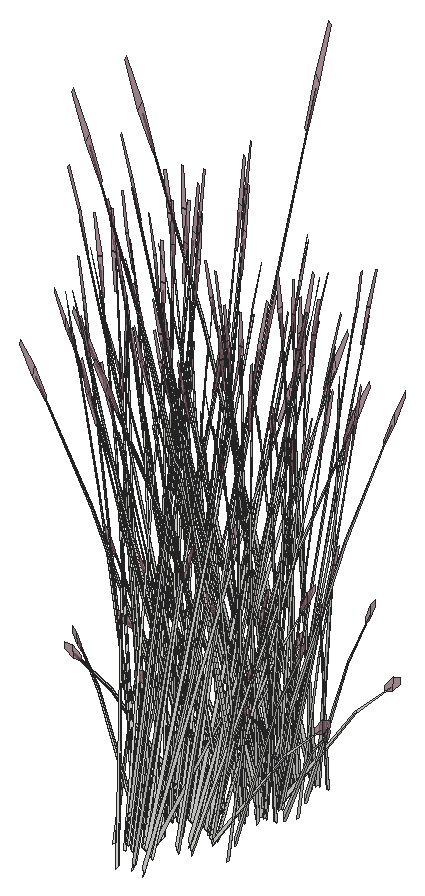
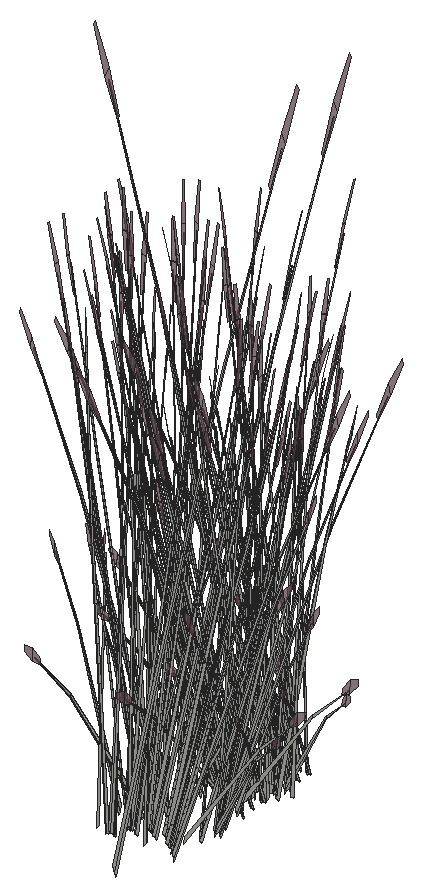
# SketchUp Ruby script. Lengths in inches.
U = 1.inch
M = Sketchup.active_model
def pt(a) = Geom::Point3d.new(a.map { |v| v * U })
def face(e, loops, mat)
  f = e.add_face(loops[0].map { |a| pt(a) })
  loops[1..].each { |l| e.add_face(l.map { |a| pt(a) }).erase! }
  f.material = f.back_material = mat if mat
  f
end
# faces: each face lists its corners as indices into pts; further lists are holes
def faces(e, pts, list, mat = nil) = list.each { |f| face(e, (f[0].is_a?(Array) ? f : [f]).map { |l| l.map { |i| pts[i] } }, mat) }
# xy, xz, yz: faces in a plane at the given z, y or x. An outline is a flat list of corners, or four numbers for a rectangle; further outlines are holes
def ring(l) = l.size == 4 ? [[l[0], l[1]], [l[2], l[1]], [l[2], l[3]], [l[0], l[3]]] : l.each_slice(2).to_a
def flat(e, list, mat, &to3) = list.each { |f| face(e, (f[0].is_a?(Array) ? f : [f]).map { |l| ring(l).map { |u, v| to3.(u, v) } }, mat) }
def xy(e, z, list, mat = nil) = flat(e, list, mat) { |x, y| [x, y, z] }
def xz(e, y, list, mat = nil) = flat(e, list, mat) { |x, z| [x, y, z] }
def yz(e, x, list, mat = nil) = flat(e, list, mat) { |y, z| [x, y, z] }
def lines(e, pts, list) = list.each { |a, b| e.add_line(pt(pts[a]), pt(pts[b])) }
# prism: a flat outline (further loops are holes) pulled along v
def prism(e, loops, v, mat = nil)
  f = face(e, loops, mat); d = Geom::Vector3d.new(v.map { |x| x * U })
  f.pushpull(f.normal.samedirection?(d) ? d.length : -d.length)
end
def box(e, o, s, mat = nil) = prism(e, [[o, [o[0] + s[0], o[1], o[2]], [o[0] + s[0], o[1] + s[1], o[2]], [o[0], o[1] + s[1], o[2]]]], [0, 0, s[2]], mat)
def at(x, y, z, deg = 0) = Geom::Transformation.translation(pt([x, y, z])) * Geom::Transformation.rotation(ORIGIN, Z_AXIS, deg.degrees)
def axes(o, x, y, z) = Geom::Transformation.new([*x, 0, *y, 0, *z, 0, *pt(o).to_a, 1])
def part(name) = M.definitions.add(name)
# library, detail: a bought-in or finely detailed component or shape, given as its bounding box
def library(name, o, s) = part(name).tap { |d| box(d.entities, o, s) }
def detail(e, o, s) = box(e.add_group.entities, o, s)
def put(e, d, t, mat = nil) = e.add_instance(d, t).tap { |i| i.material = mat if mat }
def group(e, t, mat = nil) = e.add_group.tap { |g| g.transformation = t; g.material = mat if mat }.entities
root = M.entities
M.materials.add("LightPink_Translucent").color = [144, 107, 117]
M.materials["LightPink_Translucent"].alpha = 0.75
c1 = part("blade")
p = [[2.15,0.21,22],[0,0.17,0],[0.09,0.45,0],[2.18,0.31,22],[2.29,0.31,22],[0.38,0.45,0],
  [2.48,0.24,33],[2.49,0.24,33],[2.48,0.22,33]]
faces(c1.entities,p,[[0,1,2,3],[4,5,2,3],[6,3,4,7],[8,0,3,6]])
c2 = part("seeds")
p = [[0.3,-0.1,1.38],[-0.01,-0.03,1.59],[-0.01,-0.03,0.03],[0.14,-0.07,-0.07],[0.29,-0.03,3],[0.15,0.01,3.11]]
faces(c2.entities,p,[[0,1,2,3],[1,0,4,5]],"LightPink_Translucent")
c3 = part("blade with seeds")
put(c3.entities,c1,at(0,0,0))
put(c3.entities,c2,axes([2.4,0.25,30.99],[1.5799,-0.05474,1.17369],[-0.12525,1.92788,0.29478],[-0.07173,-0.02425,1.56792]))
put(root,c3,axes([430.38,464.01,154.25],[-0.45039,-0.02337,-0.10273],[0.01231,-0.44247,-0.57019],[0.03129,-0.17041,0.8664]))
put(root,c3,axes([430.35,463.72,153.82],[0.27728,-0.24833,-0.29918],[0.26248,0.28355,0.38624],[0.03994,-0.14407,0.73904]))
put(root,c3,axes([429.54,463.34,154],[0.30197,-0.1603,0.05432],[0.1478,0.29231,0.42765],[-0.02916,-0.12885,0.65209]))
put(root,c3,axes([427.77,457.25,153.27],[0.0763,-0.16212,1.44779],[0.3201,0.3355,0.11706],[-0.1444,0.2091,0.61892]))
put(root,c3,axes([428.35,463.42,153.82],[-0.06329,-0.37991,-0.29918],[0.36182,-0.10032,0.38624],[-0.09718,-0.10887,0.73904]))
put(root,c3,axes([428.66,458.54,154],[-0.30197,0.1603,0.05432],[-0.1478,-0.29231,0.42765],[0.02916,0.12885,0.65209]))
put(root,c3,axes([427.85,458.16,153.82],[-0.27728,0.24833,-0.29918],[-0.26248,-0.28355,0.38624],[-0.03994,0.14407,0.73904]))
put(root,c3,axes([426.9,458.09,153.98],[-0.01019,0.09334,1.47793],[0.28908,0.3247,-0.23373],[-0.07568,0.15355,0.11853]))
put(root,c3,axes([427.82,457.875,154.56],[0.45039,0.02337,-0.11403],[-0.01231,0.44247,-0.63292],[-0.03129,0.17041,0.9617]))
put(root,c3,axes([431.71,461.76,153.98],[-0.03706,-0.04129,1.49853],[0.08106,-0.44261,-0.1416],[0.14596,-0.02828,0.26519]))
put(root,c3,axes([428.66,458.37,154.25],[0.40102,-0.2196,-0.10273],[0.19707,0.38974,-0.57019],[0.05291,0.16424,0.8664]))
put(root,c3,axes([426.89,459.96,153.98],[-0.06692,0.06124,1.47793],[0.00569,0.44742,-0.23373],[-0.15339,0.05818,0.11853]))
put(root,c3,axes([427.34,459.9,153.95],[-0.11102,0.42903,-0.43168],[-0.38064,-0.14706,-0.33437],[-0.15325,0.03934,0.82598]))
put(root,c3,axes([427.32,459.54,154.25],[0.20619,0.42709,-0.10273],[-0.36595,0.20988,-0.57019],[-0.15422,0.05635,0.8664]))
put(root,c3,axes([428.51,463.38,154],[0.18625,-0.29962,0.05432],[0.26523,0.17444,0.42765],[-0.08575,-0.09606,0.65209]))
put(root,c3,axes([431.39,461.39,153.32],[-0.07843,-0.39649,-0.0295],[0.37072,-0.09115,-0.13375],[0.07742,0.02514,0.44114]))
put(root,c3,axes([430.43,461.38,154.25],[0.02194,-0.47967,-0.10273],[0.41546,0.01311,-0.57019],[0.16001,0.03332,0.8664]))
put(root,c3,axes([427.57,463.97,153.27],[0.15222,0.08126,1.44779],[-0.31502,0.34091,0.11706],[-0.19634,-0.15379,0.61892]))
put(root,c3,axes([428.13,458.04,154.23],[0.29336,0.31691,-0.47917],[-0.3099,0.27755,-0.37115],[-0.04464,0.16102,0.91684]))
put(root,c3,axes([429,458.35,153.95],[0.40284,0.11824,-0.43168],[-0.13808,0.40538,-0.33437],[0.03694,0.16321,0.82598]))
put(root,c3,axes([429.23,457.51,153.27],[-0.09368,-0.15143,1.44779],[0.43286,-0.12749,0.11706],[0.09783,0.23774,0.61892]))
put(root,c3,axes([428.31,463.73,153.95],[-0.40438,0.11212,-0.43168],[-0.07074,-0.4246,-0.33437],[-0.10862,-0.12168,0.82598]))
put(root,c3,axes([430.35,463.82,154],[0.29182,0.32181,0.40553],[-0.3099,0.27755,0.33437],[0.05383,-0.15098,0.83914]))
put(root,c3,axes([428.59,463.35,154.59],[-0.2735,0.45217,-0.11506],[-0.39608,-0.2605,-0.63862],[-0.13768,-0.12775,0.97037]))
put(root,c3,axes([430.46,463.85,154],[0.33677,0.02198,0.05432],[-0.00923,0.33185,0.42765],[0.03524,-0.12712,0.65209]))
put(root,c3,axes([428.82,458.6,153.82],[-0.12355,0.36271,-0.29918],[-0.36044,-0.10579,0.38624],[0.03305,0.14603,0.73904]))
put(root,c3,axes([430.6875,464.57,153.95],[-0.10528,-0.43067,-0.43168],[0.39868,-0.07534,-0.33437],[0.11425,-0.11568,0.82598]))
put(root,c3,axes([428.04,457.9,154.51],[-0.01066,0.43628,-0.66621],[-0.44902,-0.0293,0.0804],[-0.04739,0.18483,0.94242]))
put(root,c3,axes([430.79,461.09,153.98],[0.08791,-0.00798,1.47793],[0.24113,-0.36643,-0.23373],[0.15637,0.04837,0.11853]))
put(root,c3,axes([426.87,459.04,153.98],[0.04649,-0.02848,1.49853],[0.38427,0.18941,-0.1416],[-0.00903,0.15771,0.26519]))
put(root,c3,axes([427.27,460.73,154],[-0.10163,-0.43409,0.40553],[0.39868,-0.07534,0.33437],[-0.1175,0.10209,0.83914]))
put(root,c3,axes([427.19,460.65,154],[-0.28133,-0.19836,0.05432],[0.16379,-0.28248,0.42765],[-0.0902,0.09132,0.65209]))
put(root,c3,axes([427.32,460.125,153.27],[0.14219,-0.09977,1.44779],[0.11971,0.461,0.11706],[-0.22323,0.10419,0.61892]))
put(root,c3,axes([428.46,457.59,153.27],[-0.01003,-0.18103,1.44779],[0.43473,0.12009,0.11706],[-0.02689,0.25798,0.61892]))
put(root,c3,axes([427.54,463.22,153.98],[-0.08817,-0.00333,1.47793],[-0.28072,0.33293,-0.23373],[-0.14978,-0.06803,0.11853]))
put(root,c3,axes([430.875,464.88,154.25],[-0.37908,-0.26007,-0.10273],[0.21839,-0.37663,-0.57019],[0.1071,-0.13092,0.8664]))
put(root,c3,axes([429.31,466.3,152.81],[0.35414,0.19019,1.27785],[-0.34693,0.40974,0.50532],[-0.1554,-0.24285,1.07126]))
put(root,c3,axes([428.5625,459.24,153.98],[0.05195,0.07595,1.47793],[0.41921,0.02984,-0.23373],[0.04216,0.1675,0.11853]))
put(root,c3,axes([431.81,464.77,153.98],[-0.05353,-0.00358,1.49853],[-0.22227,-0.38383,-0.1416],[0.08926,-0.1262,0.26519]))
put(root,c3,axes([426.14,460.42,153.98],[0.0523,0.01265,1.49853],[0.16179,0.41674,-0.1416],[-0.10706,0.10938,0.26519]))
put(root,c3,axes([430.69,461.34,153.82],[0.23317,0.29531,-0.29918],[-0.26625,0.27955,0.38624],[0.13527,0.04253,0.73904]))
put(root,c3,axes([430.57,461.46,154],[-0.02064,0.35866,0.05432],[-0.3116,-0.00983,0.42765],[0.11936,0.03753,0.65209]))
put(root,c3,axes([427.23,460.8125,153.82],[-0.35672,0.06741,-0.29918],[-0.09419,-0.38534,0.38624],[-0.10222,0.1035,0.73904]))
put(root,c3,axes([430.98,464.62,153.82],[0.35672,-0.06741,-0.29918],[0.09419,0.38534,0.38624],[0.10222,-0.1035,0.73904]))
put(root,c3,axes([430.6,461.34,154],[-0.30217,0.31079,0.40553],[-0.2606,-0.33005,0.33437],[0.14177,0.05733,0.83914]))
put(root,c3,axes([427.63,463.97,154],[0.02064,-0.35866,0.05432],[0.3116,0.00983,0.42765],[-0.11936,-0.03753,0.65209]))
put(root,c3,axes([427.51,464.09,153.82],[-0.23317,-0.29531,-0.29918],[0.26625,-0.27955,0.38624],[-0.13527,-0.04253,0.73904]))
put(root,c3,axes([427.89,458.51,152.84],[0.009,-0.24349,1.30391],[0.40497,0.12861,0.18019],[-0.03509,0.2595,0.61571]))
put(root,c3,axes([429.86,460.59,153.27],[-0.15222,-0.08126,1.44779],[0.31502,-0.34091,0.11706],[0.19634,0.15379,0.61892]))
put(root,c3,axes([429.88,459.52,153.78],[-0.35411,-0.24507,1.16821],[0.37391,-0.38156,0.50405],[0.11425,0.22994,1.12919]))
put(root,c3,axes([427.33,460.55,154.25],[0.37908,0.26007,-0.10273],[-0.21839,0.37663,-0.57019],[-0.1071,0.13092,0.8664]))
put(root,c3,axes([429.61,461.9,154.25],[0.2442,-0.40372,-0.10273],[0.35364,0.23259,-0.57019],[0.12293,0.11406,0.8664]))
put(root,c3,axes([431.01,464.78,154],[0.28133,0.19836,0.05432],[-0.16379,0.28248,0.42765],[0.0902,-0.09132,0.65209]))
put(root,c3,axes([428.2,467.55,153.27],[0.09368,0.15143,1.44779],[-0.43286,0.12749,0.11706],[-0.09783,-0.23774,0.61892]))
put(root,c3,axes([430.93,464.7,154],[0.10163,0.43409,0.40553],[-0.39868,0.07534,0.33437],[0.1175,-0.10209,0.83914]))
put(root,c3,axes([432.01,465.22,153.98],[0.05687,-0.07184,1.47793],[-0.07279,-0.44069,-0.23373],[0.14268,-0.08356,0.11853]))
put(root,c3,axes([427.84,460.44,153.27],[0.10236,-0.14492,1.44779],[0.25844,0.39118,0.11706],[-0.17726,0.17814,0.61892]))
put(root,c3,axes([427.52,460.86,153.95],[0.10528,0.43067,-0.43168],[-0.39868,0.07534,-0.33437],[-0.11425,0.11568,0.82598]))
put(root,c3,axes([428.91,466.55,153.98],[-0.06268,-0.06613,1.47793],[-0.4183,0.04193,-0.23373],[-0.06676,-0.15817,0.11853]))
put(root,c3,axes([427.2,463.5,153.98],[0.03038,0.04707,1.49853],[-0.14646,0.42312,-0.1416],[-0.14833,0.00306,0.26519]))
put(root,c3,axes([429.29,462.23,153.98],[0.00121,-0.0571,1.49853],[0.35119,-0.25193,-0.1416],[0.12199,0.08992,0.26519]))
put(root,c3,axes([427.75,461.58,154],[-0.33677,-0.02198,0.05432],[0.00923,-0.33185,0.42765],[-0.03524,0.12712,0.65209]))
put(root,c3,axes([427.85,461.61,154],[-0.29182,-0.32181,0.40553],[0.3099,-0.27755,0.33437],[-0.05383,0.15098,0.83914]))
put(root,c3,axes([429.9,461.7,153.95],[0.40438,-0.11212,-0.43168],[0.07074,0.4246,-0.33437],[0.10862,0.12168,0.82598]))
put(root,c3,axes([427.625,464.38,153.95],[-0.29757,0.31243,-0.43168],[-0.2606,-0.33005,-0.33437],[-0.15119,-0.04754,0.82598]))
put(root,c3,axes([427.78,464.05,154.25],[-0.02194,0.47967,-0.10273],[-0.41546,-0.01311,-0.57019],[-0.16001,-0.03332,0.8664]))
put(root,c3,axes([429.7,462.05,154],[-0.18625,0.29962,0.05432],[-0.26523,-0.17444,0.42765],[0.08575,0.09606,0.65209]))
put(root,c3,axes([430.79,467.36,153.98],[-0.00396,-0.09387,1.47793],[-0.33411,-0.2713,-0.23373],[0.05166,-0.16446,0.11853]))
put(root,c3,axes([429.39,467.34,153.82],[0.12355,-0.36271,-0.29918],[0.36044,0.10579,0.38624],[-0.03305,-0.14603,0.73904]))
put(root,c3,axes([429.66,467.82,153.27],[-0.0763,0.16212,1.44779],[-0.3201,-0.3355,0.11706],[0.1444,-0.2091,0.61892]))
put(root,c3,axes([430.7,467.02,153.98],[-0.04162,0.03603,1.49853],[-0.40776,-0.12155,-0.1416],[-0.01476,-0.15722,0.26519]))
put(root,c3,axes([430.89,465.89,154.25],[-0.20619,-0.42709,-0.10273],[0.36595,-0.20988,-0.57019],[0.15422,-0.05635,0.8664]))
put(root,c3,axes([430.87,465.53,153.95],[0.11102,-0.42903,-0.43168],[0.38064,0.14706,-0.33437],[0.15325,-0.03934,0.82598]))
put(root,c3,axes([427.25,464.71,153.27],[0.16998,-0.01068,1.44779],[-0.11276,0.46299,0.11706],[-0.24224,-0.02864,0.61892]))
put(root,c3,axes([429.78,461.96,154],[-0.4076,0.10824,0.40553],[-0.07074,-0.4246,0.33437],[0.09586,0.12514,0.83914]))
put(root,c3,axes([429.21,467.59,153.95],[-0.40284,-0.11824,-0.43168],[0.13808,-0.40538,-0.33437],[-0.03694,-0.16321,0.82598]))
put(root,c3,axes([427.77,460.79,153.27],[0.0763,-0.16212,1.44779],[0.3201,0.3355,0.11706],[-0.1444,0.2091,0.61892]))
put(root,c3,axes([430.08,467.89,153.95],[-0.29336,-0.31691,-0.43168],[0.3099,-0.27755,-0.33437],[0.04464,-0.16102,0.82598]))
put(root,c3,axes([428.49,466.33,153.98],[-0.00765,0.05653,1.49853],[-0.37706,0.20517,-0.1416],[-0.11096,-0.10488,0.26519]))
put(root,c3,axes([428.66,462.09,154],[-0.30197,0.1603,0.05432],[-0.1478,-0.29231,0.42765],[0.02916,0.12885,0.65209]))
put(root,c3,axes([427.85,461.71,153.82],[-0.27728,0.24833,-0.29918],[-0.26248,-0.28355,0.38624],[-0.03994,0.14407,0.73904]))
put(root,c3,axes([426.9,461.63,153.98],[-0.01019,0.09334,1.47793],[0.28908,0.3247,-0.23373],[-0.07568,0.15355,0.11853]))
put(root,c3,axes([427.82,461.42,154.56],[0.45039,0.02337,-0.11403],[-0.01231,0.44247,-0.63292],[-0.03129,0.17041,0.9617]))
put(root,c3,axes([428.66,461.92,154.25],[0.40102,-0.2196,-0.10273],[0.19707,0.38974,-0.57019],[0.05291,0.16424,0.8664]))
put(root,c3,axes([429.43,467.42,154],[0.4038,0.12331,0.40553],[-0.13808,0.40538,0.33437],[-0.02427,-0.15942,0.83914]))
put(root,c3,axes([429.55,467.57,154.25],[-0.40102,0.2196,-0.10273],[-0.19707,-0.38974,-0.57019],[-0.05291,-0.16424,0.8664]))
put(root,c3,axes([430.38,468.06,154.25],[-0.45039,-0.02337,-0.10273],[0.01231,-0.44247,-0.57019],[0.03129,-0.17041,0.8664]))
put(root,c3,axes([430.35,467.78,153.82],[0.27728,-0.24833,-0.29918],[0.26248,0.28355,0.38624],[0.03994,-0.14407,0.73904]))
put(root,c3,axes([429.54,467.39,154],[0.30197,-0.1603,0.05432],[0.1478,0.29231,0.42765],[-0.02916,-0.12885,0.65209]))
put(root,c3,axes([428.35,467.47,153.82],[-0.06329,-0.37991,-0.29918],[0.36182,-0.10032,0.38624],[-0.09718,-0.10887,0.73904]))
put(root,c3,axes([427.18,465.0625,154],[0.11578,-0.43006,0.40553],[0.38064,0.14706,0.33437],[-0.14969,0.02584,0.83914]))
put(root,c3,axes([427.15,464.95,154],[-0.15051,-0.3216,0.05432],[0.27447,-0.15741,0.42765],[-0.12099,0.03106,0.65209]))
put(root,c3,axes([428.13,461.59,154.23],[0.29336,0.31691,-0.47917],[-0.3099,0.27755,-0.37115],[-0.04464,0.16102,0.91684]))
put(root,c3,axes([429,461.9,153.95],[0.40284,0.11824,-0.43168],[-0.13808,0.40538,-0.33437],[0.03694,0.16321,0.82598]))
put(root,c3,axes([429.23,461.06,153.27],[-0.09368,-0.15143,1.44779],[0.43286,-0.12749,0.11706],[0.09783,0.23774,0.61892]))
put(root,c3,axes([428.82,462.14,153.82],[-0.12355,0.36271,-0.29918],[-0.36044,-0.10579,0.38624],[0.03305,0.14603,0.73904]))
put(root,c3,axes([428.51,467.4375,154],[0.18625,-0.29962,0.05432],[0.26523,0.17444,0.42765],[-0.08575,-0.09606,0.65209]))
put(root,c3,axes([431.1,465.72,153.82],[0.34057,0.13158,-0.29918],[-0.09933,0.38387,0.38624],[0.13712,-0.0352,0.73904]))
put(root,c3,axes([428.04,461.44,154.51],[-0.01066,0.43628,-0.66621],[-0.44902,-0.0293,0.0804],[-0.04739,0.18483,0.94242]))
put(root,c3,axes([427.57,468.02,153.27],[0.15222,0.08126,1.44779],[-0.31502,0.34091,0.11706],[-0.19634,-0.15379,0.61892]))
put(root,c3,axes([426.87,462.59,153.98],[0.04649,-0.02848,1.49853],[0.38427,0.18941,-0.1416],[-0.00903,0.15771,0.26519]))
put(root,c3,axes([427.1,465.11,153.82],[-0.34057,-0.13158,-0.29918],[0.09933,-0.38387,0.38624],[-0.13712,0.0352,0.73904]))
put(root,c3,axes([428.46,461.13,153.27],[-0.01003,-0.18103,1.44779],[0.43473,0.12009,0.11706],[-0.02689,0.25798,0.61892]))
put(root,c3,axes([428.31,467.78,153.95],[-0.40438,0.11212,-0.43168],[-0.07074,-0.4246,-0.33437],[-0.10862,-0.12168,0.82598]))
put(root,c3,axes([430.35,467.87,154],[0.29182,0.32181,0.40553],[-0.3099,0.27755,0.33437],[0.05383,-0.15098,0.83914]))
put(root,c3,axes([430.18,465.25,153.27],[-0.16998,0.01068,1.44779],[0.11276,-0.46299,0.11706],[0.24224,0.02864,0.61892]))
put(root,c3,axes([428.59,467.4,154.59],[-0.2735,0.45217,-0.11506],[-0.39608,-0.2605,-0.63862],[-0.13768,-0.12775,0.97037]))
put(root,c3,axes([430.46,467.9,154],[0.33677,0.02198,0.05432],[-0.00923,0.33185,0.42765],[0.03524,-0.12712,0.65209]))
put(root,c3,axes([431.05,465.88,154],[0.15051,0.3216,0.05432],[-0.27447,0.15741,0.42765],[0.12099,-0.03106,0.65209]))
put(root,c3,axes([430.6875,468.625,153.95],[-0.10528,-0.43067,-0.43168],[0.39868,-0.07534,-0.33437],[0.11425,-0.11568,0.82598]))
put(root,c3,axes([431.03,465.77,154],[-0.11578,0.43006,0.40553],[-0.38064,-0.14706,0.33437],[0.14969,-0.02584,0.83914]))
put(root,c3,axes([428.5625,462.79,153.98],[0.05195,0.07595,1.47793],[0.41921,0.02984,-0.23373],[0.04216,0.1675,0.11853]))
put(root,c3,axes([427.54,467.27,153.98],[-0.08817,-0.00333,1.47793],[-0.28072,0.33293,-0.23373],[-0.14978,-0.06803,0.11853]))
put(root,c3,axes([430.875,468.93,154.25],[-0.37908,-0.26007,-0.10273],[0.21839,-0.37663,-0.57019],[0.1071,-0.13092,0.8664]))
put(root,c3,axes([428.14,465.05,152.82],[0.11649,-0.06823,1.49584],[0.04017,0.47639,0.11706],[-0.25231,0.06321,0.53462]))
put(root,c3,axes([429.31,470.35,152.81],[0.35414,0.19019,1.27785],[-0.34693,0.40974,0.50532],[-0.1554,-0.24285,1.07126]))
put(root,c3,axes([427.89,462.06,152.84],[0.009,-0.24349,1.30391],[0.40497,0.12861,0.18019],[-0.03509,0.2595,0.61571]))
put(root,c3,axes([431.81,468.82,153.98],[-0.05353,-0.00358,1.49853],[-0.22227,-0.38383,-0.1416],[0.08926,-0.1262,0.26519]))
put(root,c3,axes([431.71,467.16,153.98],[-0.03706,-0.04129,1.49853],[0.08106,-0.44261,-0.1416],[0.14596,-0.02828,0.26519]))
put(root,c3,axes([426.89,465.37,153.98],[-0.06692,0.06124,1.47793],[0.00569,0.44742,-0.23373],[-0.15339,0.05818,0.11853]))
put(root,c3,axes([427.34,465.31,153.95],[-0.11102,0.42903,-0.43168],[-0.38064,-0.14706,-0.33437],[-0.15325,0.03934,0.82598]))
put(root,c3,axes([427.32,464.94,154.25],[0.20619,0.42709,-0.10273],[-0.36595,0.20988,-0.57019],[-0.15422,0.05635,0.8664]))
put(root,c3,axes([431.39,466.79,153.32],[-0.07843,-0.39649,-0.0295],[0.37072,-0.09115,-0.13375],[0.07742,0.02514,0.44114]))
put(root,c3,axes([430.43,466.78,154.25],[0.02194,-0.47967,-0.10273],[0.41546,0.01311,-0.57019],[0.16001,0.03332,0.8664]))
put(root,c3,axes([430.98,468.67,153.82],[0.35672,-0.06741,-0.29918],[0.09419,0.38534,0.38624],[0.10222,-0.1035,0.73904]))
put(root,c3,axes([427.63,468.03,154],[0.02064,-0.35866,0.05432],[0.3116,0.00983,0.42765],[-0.11936,-0.03753,0.65209]))
put(root,c3,axes([427.51,468.14,153.82],[-0.23317,-0.29531,-0.29918],[0.26625,-0.27955,0.38624],[-0.13527,-0.04253,0.73904]))
put(root,c3,axes([430.79,466.49,153.98],[0.08791,-0.00798,1.47793],[0.24113,-0.36643,-0.23373],[0.15637,0.04837,0.11853]))
put(root,c3,axes([427.27,466.13,154],[-0.10163,-0.43409,0.40553],[0.39868,-0.07534,0.33437],[-0.1175,0.10209,0.83914]))
